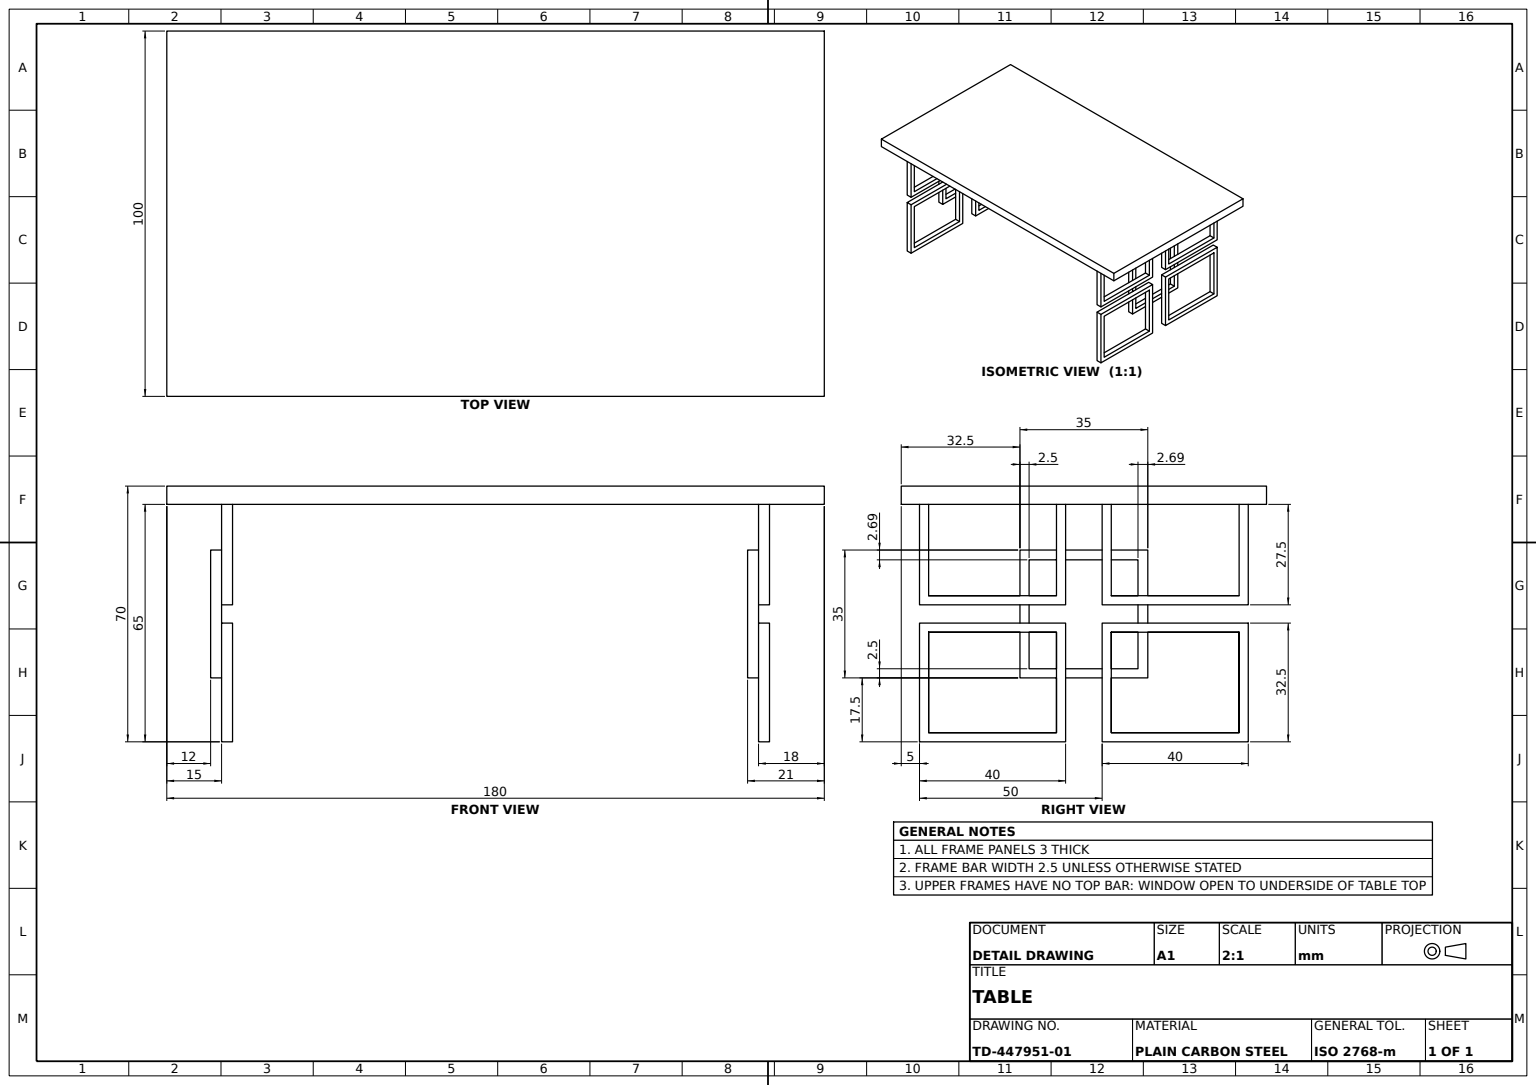
solid
v1 (2.5,65,3)
v2 (2.5,40,3)
e1 v1 v2 LINE
v3 (2.5,40,0)
e2 v3 v2 LINE
v4 (2.5,65,0)
e3 v4 v3 LINE
e4 v4 v1 LINE
face PLANE(AX(P(2.5,67.5,0),D(-1,0,0),D(0,-1,0))) rev [e1 -e2 -e3 e4]
v5 (27.5,37.5,3)
v6 (30.186202,37.5,3)
e5 v5 v6 LINE
v7 (0,37.5,3)
e6 v7 v5 LINE
v8 (0,37.5,0)
e7 v8 v7 LINE
v9 (40,37.5,0)
e8 v8 v9 LINE
v10 (40,37.5,3)
e9 v9 v10 LINE
e10 v6 v10 LINE
face PLANE(AX(P(0,37.5,0),D(0,-1,0),D(0,0,-1))) [-e5 -e6 -e7 e8 e9 -e10]
v11 (27.5,17.5,-144)
v12 (37.5,17.5,-144)
e11 v11 v12 LINE
v13 (40,17.5,-144)
e12 v12 v13 LINE
v14 (50,17.5,-144)
e13 v13 v14 LINE
v15 (52.5,17.5,-144)
e14 v14 v15 LINE
v16 (62.5,17.5,-144)
e15 v15 v16 LINE
v17 (62.5,17.5,-141)
e16 v17 v16 LINE
v18 (27.5,17.5,-141)
e17 v18 v17 LINE
e18 v18 v11 LINE
face PLANE(AX(P(27.5,17.5,-141),D(0,1,0),D(0,0,1))) rev [e11 e12 e13 e14 e15 -e16 -e17 e18]
v19 (90,0,-144)
v20 (90,32.5,-144)
e19 v19 v20 LINE
v21 (90,0,-147)
e20 v19 v21 LINE
v22 (90,32.5,-147)
e21 v21 v22 LINE
e22 v20 v22 LINE
face PLANE(AX(P(90,0,-144),D(-1,0,0),D(0,0,1))) rev [-e19 e20 e21 -e22]
v23 (90,65,-144)
v24 (87.5,65,-144)
e23 v23 v24 LINE
v25 (87.5,40,-144)
e24 v25 v24 LINE
v26 (62.5,40,-144)
e25 v26 v25 LINE
v27 (62.5,37.5,-144)
e26 v27 v26 LINE
v28 (90,37.5,-144)
e27 v27 v28 LINE
e28 v28 v23 LINE
face PLANE(AX(P(0,0,-144),D(0,0,1),D(1,0,0))) [e23 -e24 -e25 -e26 e27 e28]
v29 (27.5,52.5,-141)
e29 v29 v18 LINE
v30 (27.5,52.5,-144)
e30 v29 v30 LINE
v31 (27.5,40,-144)
e31 v30 v31 LINE
v32 (27.5,37.5,-144)
e32 v31 v32 LINE
v33 (27.5,32.5,-144)
e33 v32 v33 LINE
v34 (27.5,30,-144)
e34 v33 v34 LINE
e35 v34 v11 LINE
face PLANE(AX(P(27.5,52.5,-141),D(1,0,0),D(0,0,-1))) rev [-e29 e30 e31 e32 e33 e34 e35 -e18]
v35 (0,65,0)
e36 v35 v8 LINE
e37 v4 v35 LINE
v36 (37.5,40,0)
e38 v3 v36 LINE
v37 (37.5,65,0)
e39 v36 v37 LINE
v38 (40,65,0)
e40 v38 v37 LINE
e41 v9 v38 LINE
face PLANE(AX(P(0,0,0),D(0,0,-1),D(-1,0,0))) [-e36 -e37 e3 e38 e39 -e40 -e41 -e8]
v39 (37.5,65,-144)
v40 (37.5,65,-147)
e42 v39 v40 LINE
v41 (37.5,40,-147)
e43 v41 v40 LINE
v42 (37.5,40,-144)
e44 v42 v41 LINE
v43 (37.5,49.813798,-144)
e45 v42 v43 LINE
v44 (37.5,52.5,-144)
e46 v43 v44 LINE
e47 v44 v39 LINE
face PLANE(AX(P(37.5,67.5,-144),D(-1,0,0),D(0,0,1))) [e42 -e43 -e44 e45 e46 e47]
v45 (62.5,52.5,3)
v46 (52.5,52.5,3)
e48 v45 v46 LINE
v47 (50,52.5,3)
e49 v47 v46 LINE
v48 (40,52.5,3)
e50 v47 v48 LINE
v49 (37.5,52.5,3)
e51 v49 v48 LINE
v50 (27.5,52.5,3)
e52 v49 v50 LINE
v51 (27.5,52.5,6)
e53 v51 v50 LINE
v52 (62.5,52.5,6)
e54 v52 v51 LINE
e55 v52 v45 LINE
face PLANE(AX(P(27.5,52.5,6),D(0,-1,0),D(0,0,-1))) rev [e48 -e49 e50 -e51 e52 -e53 -e54 e55]
v53 (37.5,49.813798,3)
v54 (30.186202,49.813798,3)
e56 v53 v54 LINE
v55 (30.186202,40,3)
e57 v54 v55 LINE
v56 (27.5,40,3)
e58 v56 v55 LINE
e59 v50 v56 LINE
e60 v53 v49 LINE
face PLANE(AX(P(0,0,3),D(0,0,-1),D(-1,0,0))) [e56 e57 -e58 -e59 -e52 -e60]
v57 (37.5,65,3)
e61 v49 v57 LINE
v58 (40,65,3)
e62 v48 v58 LINE
e63 v58 v57 LINE
face PLANE(AX(P(0,0,3),D(0,0,-1),D(-1,0,0))) rev [-e61 e51 e62 e63]
v59 (40,52.5,-144)
e64 v59 v44 LINE
e65 v44 v30 LINE
v60 (62.5,52.5,-141)
e66 v60 v29 LINE
v61 (62.5,52.5,-144)
e67 v60 v61 LINE
v62 (52.5,52.5,-144)
e68 v61 v62 LINE
v63 (50,52.5,-144)
e69 v62 v63 LINE
e70 v63 v59 LINE
face PLANE(AX(P(27.5,52.5,-141),D(0,-1,0),D(0,0,-1))) rev [e64 e65 -e30 -e66 e67 e68 e69 e70]
v64 (50,37.5,-147)
v65 (90,37.5,-147)
e71 v64 v65 LINE
e72 v28 v65 LINE
v66 (60,37.5,-144)
e73 v66 v27 LINE
v67 (50,37.5,-144)
e74 v67 v66 LINE
e75 v67 v64 LINE
face PLANE(AX(P(50,37.5,-144),D(0,1,0),D(0,0,1))) rev [e71 -e72 -e27 -e73 -e74 e75]
v68 (30.186202,40,-144)
e76 v68 v42 LINE
v69 (30.186202,37.5,-144)
e77 v68 v69 LINE
v70 (40,37.5,-144)
e78 v69 v70 LINE
v71 (40,49.813798,-144)
e79 v70 v71 LINE
e80 v71 v43 LINE
face PLANE(AX(P(0,0,-144),D(0,0,1),D(1,0,0))) [-e45 -e76 e77 e78 e79 e80]
v72 (87.5,2.5,3)
v73 (87.5,30,3)
e81 v72 v73 LINE
v74 (87.5,30,0)
e82 v74 v73 LINE
v75 (87.5,2.5,0)
e83 v75 v74 LINE
e84 v75 v72 LINE
face PLANE(AX(P(87.5,30,0),D(1,0,0),D(0,0,-1))) rev [e81 -e82 -e83 e84]
v76 (37.5,40,3)
e85 v36 v76 LINE
e86 v2 v56 LINE
e87 v55 v76 LINE
face PLANE(AX(P(2.5,40,0),D(0,-1,0),D(0,0,-1))) rev [-e85 -e38 e2 e86 e58 e87]
v77 (0,32.5,3)
v78 (0,32.5,0)
e88 v77 v78 LINE
v79 (27.5,32.5,3)
e89 v79 v77 LINE
v80 (30.186202,32.5,3)
e90 v80 v79 LINE
v81 (40,32.5,3)
e91 v81 v80 LINE
v82 (40,32.5,0)
e92 v81 v82 LINE
e93 v82 v78 LINE
face PLANE(AX(P(0,32.5,3),D(0,-1,0),D(0,0,-1))) rev [-e88 -e89 -e90 -e91 e92 e93]
v83 (52.5,20,-144)
e94 v83 v15 LINE
v84 (52.5,2.5,-144)
e95 v15 v84 LINE
v85 (52.5,2.5,-147)
e96 v84 v85 LINE
v86 (52.5,30,-147)
e97 v86 v85 LINE
v87 (52.5,30,-144)
e98 v87 v86 LINE
e99 v87 v83 LINE
face PLANE(AX(P(52.5,30,-144),D(1,0,0),D(0,0,-1))) [e94 e95 e96 -e97 -e98 e99]
v88 (2.5,30,0)
v89 (2.5,2.5,0)
e100 v88 v89 LINE
v90 (2.5,30,3)
e101 v88 v90 LINE
v91 (2.5,2.5,3)
e102 v90 v91 LINE
e103 v89 v91 LINE
face PLANE(AX(P(2.5,30,0),D(-1,0,0),D(0,-1,0))) rev [-e100 e101 e102 -e103]
v92 (60,49.813798,-141)
v93 (60,49.813798,-144)
e104 v92 v93 LINE
v94 (30.186202,49.813798,-141)
e105 v92 v94 LINE
v95 (30.186202,49.813798,-144)
e106 v94 v95 LINE
e107 v43 v95 LINE
v96 (50,49.813798,-144)
e108 v96 v71 LINE
v97 (52.5,49.813798,-144)
e109 v97 v96 LINE
e110 v93 v97 LINE
face PLANE(AX(P(30.186202,49.813798,-141),D(0,-1,0),D(0,0,-1))) [-e104 e105 e106 -e107 -e80 -e108 -e109 -e110]
v98 (87.5,2.5,-144)
v99 (87.5,2.5,-147)
e111 v98 v99 LINE
e112 v85 v99 LINE
e113 v84 v98 LINE
face PLANE(AX(P(52.5,2.5,-144),D(0,1,0),D(0,0,1))) [e111 -e112 -e96 e113]
v100 (50,20,-144)
e114 v100 v83 LINE
v101 (60,30,-144)
e115 v101 v87 LINE
v102 (60,32.5,-144)
e116 v101 v102 LINE
v103 (50,32.5,-144)
e117 v102 v103 LINE
e118 v103 v100 LINE
face PLANE(AX(P(0,0,-144),D(0,0,1),D(1,0,0))) [e114 -e99 -e115 e116 e117 e118]
v104 (37.5,17.5,3)
v105 (40,17.5,3)
e119 v104 v105 LINE
v106 (50,17.5,3)
e120 v105 v106 LINE
v107 (52.5,17.5,3)
e121 v106 v107 LINE
v108 (62.5,17.5,3)
e122 v107 v108 LINE
v109 (62.5,17.5,6)
e123 v109 v108 LINE
v110 (27.5,17.5,6)
e124 v110 v109 LINE
v111 (27.5,17.5,3)
e125 v110 v111 LINE
e126 v111 v104 LINE
face PLANE(AX(P(27.5,17.5,6),D(0,1,0),D(0,0,1))) rev [e119 e120 e121 e122 -e123 -e124 e125 e126]
v112 (2.5,65,-144)
v113 (2.5,40,-144)
e127 v112 v113 LINE
v114 (2.5,40,-147)
e128 v113 v114 LINE
v115 (2.5,65,-147)
e129 v115 v114 LINE
e130 v115 v112 LINE
face PLANE(AX(P(2.5,67.5,-144),D(1,0,0),D(0,0,-1))) [e127 e128 -e129 e130]
v116 (52.5,40,3)
v117 (60,40,3)
e131 v116 v117 LINE
v118 (62.5,40,3)
e132 v117 v118 LINE
v119 (87.5,40,3)
e133 v118 v119 LINE
v120 (87.5,40,0)
e134 v120 v119 LINE
v121 (52.5,40,0)
e135 v121 v120 LINE
e136 v121 v116 LINE
face PLANE(AX(P(52.5,40,0),D(0,-1,0),D(0,0,-1))) rev [e131 e132 e133 -e134 -e135 e136]
v122 (95,70,-162)
v123 (-5,70,-162)
e137 v122 v123 LINE
v124 (-5,70,18)
e138 v123 v124 LINE
v125 (95,70,18)
e139 v124 v125 LINE
e140 v125 v122 LINE
face PLANE(AX(P(0,70,0),D(0,1,0),D(0,0,1))) [e137 e138 e139 e140]
v126 (2.5,30,-144)
v127 (2.5,30,-147)
e141 v126 v127 LINE
v128 (37.5,30,-147)
e142 v128 v127 LINE
v129 (37.5,30,-144)
e143 v129 v128 LINE
v130 (30.186202,30,-144)
e144 v129 v130 LINE
e145 v130 v34 LINE
e146 v34 v126 LINE
face PLANE(AX(P(2.5,30,-144),D(0,-1,0),D(0,0,-1))) [e141 -e142 -e143 e144 e145 e146]
e147 v100 v14 LINE
v131 (50,32.5,-147)
e148 v103 v131 LINE
v132 (50,0,-147)
e149 v131 v132 LINE
v133 (50,0,-144)
e150 v133 v132 LINE
e151 v14 v133 LINE
face PLANE(AX(P(50,0,-144),D(1,0,0),D(0,0,-1))) rev [-e147 -e118 e148 e149 -e150 -e151]
v134 (40,37.5,-147)
e152 v70 v134 LINE
v135 (40,65,-147)
e153 v134 v135 LINE
v136 (40,65,-144)
e154 v136 v135 LINE
e155 v59 v136 LINE
e156 v71 v59 LINE
face PLANE(AX(P(40,37.5,-144),D(-1,0,0),D(0,0,1))) rev [-e79 e152 e153 -e154 -e155 -e156]
v137 (27.5,30,3)
e157 v137 v111 LINE
e158 v51 v110 LINE
e159 v5 v56 LINE
e160 v5 v79 LINE
e161 v79 v137 LINE
face PLANE(AX(P(27.5,17.5,6),D(1,0,0),D(0,0,-1))) rev [e157 -e125 -e158 e53 e59 -e159 e160 e161]
v138 (30.186202,20,6)
v139 (60,20,6)
e162 v138 v139 LINE
v140 (30.186202,49.813798,6)
e163 v140 v138 LINE
v141 (60,49.813798,6)
e164 v141 v140 LINE
e165 v139 v141 LINE
e166 v109 v52 LINE
face PLANE(AX(P(0,0,6),D(0,0,-1),D(-1,0,0))) rev [-e162 -e163 -e164 -e165] [e54 e158 e124 e166]
v142 (60,20,-144)
e167 v83 v142 LINE
v143 (40,20,-144)
e168 v143 v100 LINE
v144 (37.5,20,-144)
e169 v144 v143 LINE
v145 (30.186202,20,-144)
e170 v145 v144 LINE
v146 (30.186202,20,-141)
e171 v146 v145 LINE
v147 (60,20,-141)
e172 v146 v147 LINE
e173 v147 v142 LINE
face PLANE(AX(P(30.186202,20,-141),D(0,1,0),D(0,0,1))) [-e167 -e114 -e168 -e169 -e170 -e171 e172 e173]
e174 v142 v101 LINE
v148 (62.5,30,-144)
e175 v148 v101 LINE
e176 v16 v148 LINE
face PLANE(AX(P(0,0,-144),D(0,0,1),D(1,0,0))) rev [-e15 -e94 e167 e174 -e175 -e176]
v149 (90,0,0)
v150 (90,0,3)
e177 v149 v150 LINE
v151 (90,32.5,0)
e178 v149 v151 LINE
v152 (90,32.5,3)
e179 v151 v152 LINE
e180 v150 v152 LINE
face PLANE(AX(P(90,32.5,0),D(1,0,0),D(0,0,-1))) [-e177 e178 e179 -e180]
v153 (52.5,30,0)
v154 (52.5,2.5,0)
e181 v153 v154 LINE
v155 (52.5,30,3)
e182 v153 v155 LINE
v156 (52.5,20,3)
e183 v155 v156 LINE
e184 v156 v107 LINE
v157 (52.5,2.5,3)
e185 v107 v157 LINE
e186 v154 v157 LINE
face PLANE(AX(P(52.5,30,0),D(-1,0,0),D(0,-1,0))) rev [-e181 e182 e183 e184 e185 -e186]
v158 (52.5,40,-144)
v159 (52.5,40,-147)
e187 v158 v159 LINE
v160 (52.5,65,-147)
e188 v160 v159 LINE
v161 (52.5,65,-144)
e189 v160 v161 LINE
e190 v161 v62 LINE
e191 v62 v97 LINE
e192 v97 v158 LINE
face PLANE(AX(P(52.5,67.5,-144),D(1,0,0),D(0,0,-1))) [e187 -e188 e189 e190 e191 e192]
v162 (62.5,32.5,3)
e193 v152 v162 LINE
v163 (62.5,30,3)
e194 v163 v162 LINE
e195 v73 v163 LINE
e196 v157 v72 LINE
v164 (50,0,3)
e197 v106 v164 LINE
e198 v164 v150 LINE
face PLANE(AX(P(0,0,3),D(0,0,1),D(1,0,0))) [e180 e193 -e194 -e195 -e81 -e196 -e185 -e121 e197 e198]
v165 (2.5,2.5,-144)
v166 (2.5,2.5,-147)
e199 v165 v166 LINE
v167 (37.5,2.5,-144)
e200 v165 v167 LINE
v168 (37.5,2.5,-147)
e201 v167 v168 LINE
e202 v166 v168 LINE
face PLANE(AX(P(2.5,2.5,-144),D(0,1,0),D(0,0,1))) [-e199 e200 e201 -e202]
v169 (30.186202,32.5,-144)
e203 v169 v33 LINE
e204 v32 v69 LINE
e205 v69 v169 LINE
face PLANE(AX(P(0,0,-144),D(0,0,1),D(1,0,0))) rev [e203 -e33 e204 e205]
v170 (87.5,40,-147)
v171 (87.5,65,-147)
e206 v170 v171 LINE
e207 v25 v170 LINE
e208 v24 v171 LINE
face PLANE(AX(P(87.5,67.5,-144),D(-1,0,0),D(0,0,1))) [-e206 -e207 e24 e208]
v172 (0,65,3)
e209 v35 v172 LINE
e210 v1 v172 LINE
e211 v58 v38 LINE
e212 v57 v37 LINE
v173 (-5,65,18)
v174 (95,65,18)
e213 v173 v174 LINE
v175 (-5,65,-162)
e214 v175 v173 LINE
v176 (95,65,-162)
e215 v176 v175 LINE
e216 v174 v176 LINE
v177 (0,65,-147)
v178 (0,65,-144)
e217 v177 v178 LINE
e218 v112 v178 LINE
e219 v115 v177 LINE
v179 (90,65,-147)
e220 v23 v179 LINE
e221 v179 v171 LINE
v180 (87.5,65,3)
v181 (87.5,65,0)
e222 v180 v181 LINE
v182 (90,65,3)
e223 v182 v180 LINE
v183 (90,65,0)
e224 v182 v183 LINE
e225 v183 v181 LINE
v184 (50,65,-147)
e226 v160 v184 LINE
v185 (50,65,-144)
e227 v184 v185 LINE
e228 v161 v185 LINE
e229 v136 v39 LINE
e230 v135 v40 LINE
v186 (52.5,65,0)
v187 (50,65,0)
e231 v186 v187 LINE
v188 (50,65,3)
e232 v187 v188 LINE
v189 (52.5,65,3)
e233 v189 v188 LINE
e234 v186 v189 LINE
face PLANE(AX(P(0,65,0),D(0,-1,0),D(0,0,-1))) [-e4 e37 e209 -e210] [-e63 e211 e40 -e212] [-e213 -e214 -e215 -e216] [e217 -e218 -e130 e219] [e220 e221 -e208 -e23] [-e222 -e223 e224 e225] [-e189 e226 e227 -e228] [-e42 -e229 e154 e230] [e231 e232 -e233 -e234]
e235 v94 v146 LINE
e236 v130 v145 LINE
e237 v169 v130 LINE
e238 v95 v68 LINE
face PLANE(AX(P(30.186202,49.813798,-141),D(1,0,0),D(0,0,-1))) [-e106 e235 e171 -e236 -e237 -e205 -e77 -e238]
v190 (37.5,2.5,0)
e239 v89 v190 LINE
v191 (37.5,30,0)
e240 v190 v191 LINE
e241 v191 v88 LINE
v192 (40,0,0)
e242 v192 v82 LINE
v193 (0,0,0)
e243 v193 v192 LINE
e244 v78 v193 LINE
face PLANE(AX(P(0,0,0),D(0,0,-1),D(-1,0,0))) [e100 e239 e240 e241] [-e242 -e243 -e244 -e93]
v194 (0,0,3)
e245 v77 v194 LINE
v195 (40,0,3)
e246 v194 v195 LINE
e247 v195 v105 LINE
v196 (37.5,2.5,3)
e248 v196 v104 LINE
e249 v91 v196 LINE
e250 v137 v90 LINE
face PLANE(AX(P(0,0,3),D(0,0,-1),D(-1,0,0))) rev [-e161 e89 e245 e246 e247 -e119 -e248 -e249 -e102 -e250]
e251 v195 v192 LINE
e252 v194 v193 LINE
face PLANE(AX(P(0,0,3),D(0,1,0),D(0,0,1))) rev [e243 -e251 -e246 e252]
e253 v175 v123 LINE
e254 v176 v122 LINE
face PLANE(AX(P(-5,65,-162),D(0,0,-1),D(-1,0,0))) [e253 -e137 -e254 e215]
e255 v6 v80 LINE
face PLANE(AX(P(0,0,3),D(0,0,-1),D(-1,0,0))) [e90 -e160 e5 e255]
v197 (50,49.813798,3)
v198 (40,49.813798,3)
e256 v197 v198 LINE
e257 v198 v48 LINE
e258 v47 v197 LINE
face PLANE(AX(P(0,0,3),D(0,0,-1),D(-1,0,0))) [e256 e257 -e50 e258]
v199 (0,37.5,-144)
v200 (0,37.5,-147)
e259 v199 v200 LINE
e260 v178 v199 LINE
e261 v177 v200 LINE
face PLANE(AX(P(0,37.5,-144),D(1,0,0),D(0,0,-1))) rev [-e259 -e260 -e217 e261]
e262 v190 v196 LINE
face PLANE(AX(P(2.5,2.5,0),D(0,-1,0),D(0,0,-1))) rev [-e239 e103 e249 -e262]
v201 (40,20,3)
e263 v105 v201 LINE
v202 (50,20,3)
e264 v201 v202 LINE
e265 v202 v106 LINE
face PLANE(AX(P(0,0,3),D(0,0,-1),D(-1,0,0))) [-e120 e263 e264 e265]
e266 v10 v198 LINE
face PLANE(AX(P(40,37.5,0),D(1,0,0),D(0,0,-1))) [-e9 e41 -e211 -e62 -e257 -e266]
v203 (90,37.5,0)
e267 v203 v183 LINE
v204 (50,37.5,0)
e268 v204 v203 LINE
e269 v187 v204 LINE
e270 v186 v121 LINE
e271 v120 v181 LINE
face PLANE(AX(P(0,0,0),D(0,0,-1),D(-1,0,0))) [-e267 -e268 -e269 -e231 e270 e135 e271 -e225]
v205 (37.5,20,3)
e272 v104 v205 LINE
v206 (37.5,30,3)
e273 v205 v206 LINE
e274 v191 v206 LINE
face PLANE(AX(P(37.5,30,0),D(1,0,0),D(0,0,-1))) rev [e262 e248 e272 e273 -e274 -e240]
e275 v13 v143 LINE
face PLANE(AX(P(0,0,-144),D(0,0,1),D(1,0,0))) rev [e275 e168 e147 -e13]
v207 (50,37.5,3)
v208 (60,37.5,3)
e276 v207 v208 LINE
e277 v204 v207 LINE
v209 (90,37.5,3)
e278 v203 v209 LINE
v210 (62.5,37.5,3)
e279 v210 v209 LINE
e280 v208 v210 LINE
face PLANE(AX(P(50,37.5,0),D(0,-1,0),D(0,0,-1))) [-e276 -e277 e268 e278 -e279 -e280]
e281 v209 v182 LINE
face PLANE(AX(P(90,37.5,0),D(1,0,0),D(0,1,0))) [-e224 -e281 -e278 e267]
v211 (60,40,-144)
e282 v211 v26 LINE
e283 v211 v93 LINE
e284 v26 v61 LINE
face PLANE(AX(P(0,0,-144),D(0,0,1),D(1,0,0))) rev [-e282 e283 e110 -e191 -e68 -e284]
e285 v201 v81 LINE
face PLANE(AX(P(40,0,3),D(-1,0,0),D(0,0,1))) rev [-e263 -e247 e251 e242 -e92 -e285]
e286 v63 v96 LINE
face PLANE(AX(P(0,0,-144),D(0,0,1),D(1,0,0))) rev [e286 e108 e156 -e70]
v212 (30.186202,30,3)
e287 v212 v137 LINE
v213 (30.186202,20,3)
e288 v212 v213 LINE
e289 v213 v205 LINE
face PLANE(AX(P(0,0,3),D(0,0,-1),D(-1,0,0))) [-e126 -e157 -e287 e288 e289 -e272]
e290 v113 v31 LINE
e291 v199 v32 LINE
face PLANE(AX(P(0,0,-144),D(0,0,1),D(1,0,0))) [-e32 -e290 -e127 e218 e260 e291]
v214 (62.5,32.5,-144)
e292 v214 v27 LINE
e293 v214 v102 LINE
e294 v102 v66 LINE
face PLANE(AX(P(0,0,-144),D(0,0,1),D(1,0,0))) rev [-e292 e293 e294 e73]
e295 v133 v19 LINE
e296 v20 v214 LINE
e297 v148 v214 LINE
v215 (87.5,30,-144)
e298 v215 v148 LINE
e299 v98 v215 LINE
face PLANE(AX(P(0,0,-144),D(0,0,1),D(1,0,0))) [e151 e295 e19 e296 -e297 -e298 -e299 -e113 -e95 -e14]
e300 v114 v41 LINE
e301 v31 v68 LINE
face PLANE(AX(P(2.5,40,-144),D(0,1,0),D(0,0,1))) [-e300 -e128 e290 e301 e76 e44]
e302 v206 v212 LINE
face PLANE(AX(P(2.5,30,0),D(0,1,0),D(0,0,1))) rev [-e101 -e241 e274 e302 e287 e250]
face PLANE(AX(P(0,0,3),D(1,0,0),D(0,0,-1))) rev [-e245 e88 e244 -e252]
e303 v172 v7 LINE
face PLANE(AX(P(0,37.5,0),D(-1,0,0),D(0,0,1))) [-e303 -e209 e36 e7]
v216 (40,0,-144)
e304 v216 v13 LINE
v217 (40,0,-147)
e305 v216 v217 LINE
v218 (40,32.5,-147)
e306 v217 v218 LINE
v219 (40,32.5,-144)
e307 v219 v218 LINE
e308 v143 v219 LINE
face PLANE(AX(P(40,32.5,-144),D(-1,0,0),D(0,0,1))) rev [-e275 -e304 e305 e306 -e307 -e308]
e309 v65 v179 LINE
face PLANE(AX(P(90,70,-144),D(-1,0,0),D(0,0,1))) rev [-e220 -e28 e72 e309]
e310 v198 v53 LINE
v220 (52.5,49.813798,3)
e311 v220 v197 LINE
v221 (60,49.813798,3)
e312 v221 v220 LINE
e313 v141 v221 LINE
e314 v140 v54 LINE
face PLANE(AX(P(30.186202,49.813798,6),D(0,-1,0),D(0,0,-1))) [-e56 -e310 -e256 -e311 -e312 -e313 e164 e314]
v222 (0,0,-144)
e315 v222 v216 LINE
e316 v167 v12 LINE
e317 v126 v165 LINE
v223 (0,32.5,-144)
e318 v33 v223 LINE
e319 v223 v222 LINE
face PLANE(AX(P(0,0,-144),D(0,0,1),D(1,0,0))) [e315 e304 -e12 -e316 -e200 -e317 -e146 -e34 e318 e319]
v224 (50,32.5,0)
v225 (50,0,0)
e320 v224 v225 LINE
e321 v151 v224 LINE
e322 v225 v149 LINE
e323 v154 v75 LINE
e324 v74 v153 LINE
face PLANE(AX(P(0,0,0),D(0,0,1),D(1,0,0))) rev [-e320 -e321 -e178 -e322] [e181 e323 e83 e324]
v226 (60,32.5,3)
v227 (50,32.5,3)
e325 v226 v227 LINE
e326 v227 v202 LINE
e327 v202 v156 LINE
v228 (60,30,3)
e328 v228 v155 LINE
e329 v228 v226 LINE
face PLANE(AX(P(0,0,3),D(0,0,1),D(1,0,0))) [e325 e326 e327 -e183 -e328 e329]
e330 v224 v227 LINE
e331 v162 v226 LINE
face PLANE(AX(P(50,32.5,0),D(0,1,0),D(0,0,1))) [e321 e330 -e325 -e331 -e193 -e179]
e332 v108 v163 LINE
e333 v162 v210 LINE
e334 v118 v210 LINE
e335 v118 v45 LINE
face PLANE(AX(P(62.5,17.5,6),D(-1,0,0),D(0,0,1))) rev [e123 e332 e194 e333 -e334 e335 -e55 -e166]
e336 v17 v60 LINE
face PLANE(AX(P(62.5,52.5,-141),D(-1,0,0),D(0,0,1))) rev [e284 -e67 -e336 e16 e176 e297 e292 e26]
v229 (0,32.5,-147)
v230 (0,0,-147)
e337 v229 v230 LINE
e338 v222 v230 LINE
e339 v223 v229 LINE
face PLANE(AX(P(0,32.5,-144),D(1,0,0),D(0,0,-1))) rev [e337 -e338 -e319 e339]
e340 v188 v47 LINE
e341 v197 v207 LINE
face PLANE(AX(P(50,37.5,0),D(-1,0,0),D(0,0,1))) [-e258 -e340 -e232 e269 e277 -e341]
e342 v117 v221 LINE
e343 v46 v220 LINE
face PLANE(AX(P(0,0,3),D(0,0,-1),D(-1,0,0))) [-e335 -e132 e342 e312 -e343 -e48]
v231 (87.5,30,-147)
e344 v231 v86 LINE
e345 v215 v231 LINE
face PLANE(AX(P(52.5,30,-144),D(0,-1,0),D(0,0,-1))) [e175 e115 e98 -e344 -e345 e298]
e346 v99 v231 LINE
face PLANE(AX(P(87.5,30,-144),D(-1,0,0),D(0,0,1))) [-e111 e299 e345 -e346]
e347 v174 v125 LINE
face PLANE(AX(P(95,65,-162),D(1,0,0),D(0,0,-1))) [e216 e254 -e140 -e347]
e348 v147 v92 LINE
face PLANE(AX(P(0,0,-141),D(0,0,1),D(1,0,0))) [e17 e336 e66 e29] [-e172 -e235 -e105 -e348]
face PLANE(AX(P(0,0,3),D(0,0,-1),D(-1,0,0))) rev [e303 e6 e159 -e86 -e1 e210]
e349 v189 v46 LINE
e350 v220 v116 LINE
face PLANE(AX(P(52.5,67.5,0),D(-1,0,0),D(0,0,1))) rev [e349 e343 e350 -e136 -e270 e234]
face PLANE(AX(P(0,0,-144),D(0,0,1),D(1,0,0))) [e155 e229 -e47 -e64]
e351 v12 v144 LINE
face PLANE(AX(P(0,0,-144),D(0,0,1),D(1,0,0))) rev [-e145 e236 e170 -e351 -e11 -e35]
e352 v173 v124 LINE
face PLANE(AX(P(95,65,18),D(0,0,1),D(1,0,0))) [-e352 e213 e347 -e139]
e353 v132 v21 LINE
face PLANE(AX(P(90,0,-144),D(0,1,0),D(0,0,1))) rev [e150 e353 -e20 -e295]
face PLANE(AX(P(0,0,3),D(0,0,-1),D(-1,0,0))) rev [e233 e340 e49 -e349]
face PLANE(AX(P(52.5,2.5,0),D(0,-1,0),D(0,0,-1))) rev [-e84 -e323 e186 e196]
e354 v127 v166 LINE
e355 v168 v128 LINE
e356 v218 v229 LINE
e357 v230 v217 LINE
face PLANE(AX(P(0,0,-147),D(0,0,1),D(1,0,0))) rev [e142 e354 e202 e355] [-e337 -e356 -e306 -e357]
e358 v205 v201 LINE
e359 v80 v212 LINE
face PLANE(AX(P(0,0,3),D(0,0,-1),D(-1,0,0))) rev [e358 e285 e91 e359 -e302 -e273]
e360 v185 v63 LINE
face PLANE(AX(P(0,0,-144),D(0,0,1),D(1,0,0))) [-e190 e228 e360 -e69]
e361 v138 v213 LINE
v232 (60,20,3)
e362 v139 v232 LINE
e363 v156 v232 LINE
face PLANE(AX(P(30.186202,20,6),D(0,1,0),D(0,0,1))) [-e264 -e358 -e289 -e361 e162 e362 -e363 -e327]
e364 v6 v55 LINE
e365 v76 v53 LINE
face PLANE(AX(P(0,0,3),D(0,0,-1),D(-1,0,0))) rev [-e87 -e364 e10 e266 e310 -e365]
face PLANE(AX(P(0,0,-144),D(0,1,0),D(0,0,1))) rev [-e305 -e315 e338 e357]
e366 v119 v180 LINE
face PLANE(AX(P(87.5,67.5,0),D(1,0,0),D(0,0,-1))) rev [e134 e366 e222 -e271]
e367 v184 v64 LINE
e368 v96 v67 LINE
face PLANE(AX(P(50,70,-144),D(1,0,0),D(0,0,-1))) rev [-e286 -e360 -e227 e367 -e75 -e368]
e369 v22 v131 LINE
face PLANE(AX(P(0,0,-147),D(0,0,1),D(1,0,0))) rev [e97 e112 e346 e344] [-e353 -e149 -e369 -e21]
face PLANE(AX(P(90,32.5,-144),D(0,-1,0),D(0,0,-1))) rev [-e296 e22 e369 -e148 -e117 -e293]
face PLANE(AX(P(0,0,3),D(0,0,-1),D(-1,0,0))) rev [e334 e279 e281 e223 -e366 -e133]
e370 v117 v208 LINE
face PLANE(AX(P(0,0,3),D(0,0,-1),D(-1,0,0))) rev [-e350 e311 e341 e276 -e370 -e131]
face PLANE(AX(P(2.5,30,-144),D(1,0,0),D(0,0,-1))) [e199 -e354 -e141 e317]
e371 v232 v228 LINE
e372 v163 v228 LINE
face PLANE(AX(P(0,0,3),D(0,0,-1),D(-1,0,0))) [e371 -e372 -e332 -e122 -e184 e363]
e373 v144 v129 LINE
e374 v219 v169 LINE
face PLANE(AX(P(0,0,-144),D(0,0,1),D(1,0,0))) [e237 -e144 -e373 e169 e308 e374]
face PLANE(AX(P(37.5,30,-144),D(-1,0,0),D(0,0,1))) [-e355 -e201 e316 e351 e373 e143]
e375 v225 v164 LINE
face PLANE(AX(P(50,0,0),D(0,-1,0),D(0,0,-1))) [-e198 -e375 e322 e177]
face PLANE(AX(P(37.5,67.5,0),D(1,0,0),D(0,0,-1))) rev [e60 e61 e212 -e39 e85 e365]
face PLANE(AX(P(0,32.5,-144),D(0,-1,0),D(0,0,-1))) rev [-e318 -e203 -e374 e307 e356 -e339]
e376 v66 v211 LINE
face PLANE(AX(P(60,49.813798,-141),D(-1,0,0),D(0,0,1))) [-e376 -e294 -e116 -e174 -e173 e348 e104 -e283]
e377 v226 v208 LINE
face PLANE(AX(P(0,0,3),D(0,0,-1),D(-1,0,0))) [e331 e377 e280 -e333]
face PLANE(AX(P(-5,65,0),D(-1,0,0),D(0,0,1))) [e352 -e138 -e253 e214]
face PLANE(AX(P(50,32.5,0),D(-1,0,0),D(0,-1,0))) [-e265 -e326 -e330 e320 e375 -e197]
face PLANE(AX(P(30.186202,49.813798,6),D(1,0,0),D(0,1,0))) [-e57 -e314 e163 e361 -e288 -e359 -e255 e364]
face PLANE(AX(P(0,0,-144),D(0,0,1),D(1,0,0))) rev [-e65 -e46 e107 e238 -e301 -e31]
e378 v200 v134 LINE
face PLANE(AX(P(40,37.5,-144),D(0,1,0),D(0,0,1))) rev [e378 -e152 -e78 -e204 -e291 e259]
e379 v158 v211 LINE
face PLANE(AX(P(0,0,-144),D(0,0,1),D(1,0,0))) [e376 -e379 -e192 e109 e368 e74]
e380 v159 v170 LINE
face PLANE(AX(P(52.5,40,-144),D(0,1,0),D(0,0,1))) [-e187 e379 e282 e25 e207 -e380]
face PLANE(AX(P(60,49.813798,6),D(-1,0,0),D(0,-1,0))) [-e329 -e371 -e362 e165 e313 -e342 e370 -e377]
face PLANE(AX(P(0,0,-147),D(0,0,1),D(1,0,0))) rev [e300 e43 -e230 -e153 -e378 -e261 -e219 e129]
face PLANE(AX(P(0,0,-147),D(0,0,1),D(1,0,0))) rev [e188 e380 e206 -e221 -e309 -e71 -e367 -e226]
face PLANE(AX(P(52.5,30,0),D(0,1,0),D(0,0,1))) rev [e82 e195 e372 e328 -e182 -e324]
